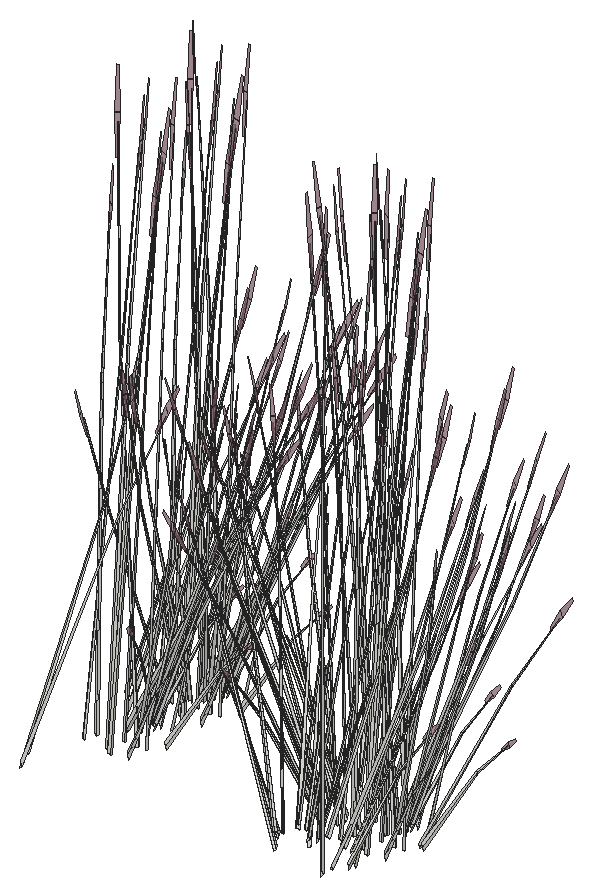
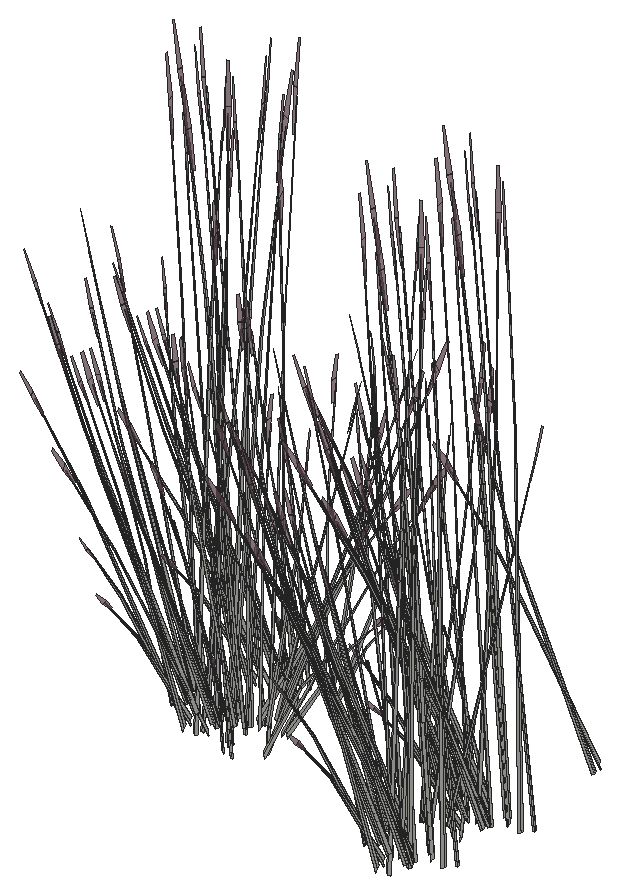
# SketchUp Ruby script. Lengths in inches.
U = 1.inch
M = Sketchup.active_model
def pt(a) = Geom::Point3d.new(a.map { |v| v * U })
def face(e, loops, mat)
  f = e.add_face(loops[0].map { |a| pt(a) })
  loops[1..].each { |l| e.add_face(l.map { |a| pt(a) }).erase! }
  f.material = f.back_material = mat if mat
  f
end
# faces: each face lists its corners as indices into pts; further lists are holes
def faces(e, pts, list, mat = nil) = list.each { |f| face(e, (f[0].is_a?(Array) ? f : [f]).map { |l| l.map { |i| pts[i] } }, mat) }
# xy, xz, yz: faces in a plane at the given z, y or x. An outline is a flat list of corners, or four numbers for a rectangle; further outlines are holes
def ring(l) = l.size == 4 ? [[l[0], l[1]], [l[2], l[1]], [l[2], l[3]], [l[0], l[3]]] : l.each_slice(2).to_a
def flat(e, list, mat, &to3) = list.each { |f| face(e, (f[0].is_a?(Array) ? f : [f]).map { |l| ring(l).map { |u, v| to3.(u, v) } }, mat) }
def xy(e, z, list, mat = nil) = flat(e, list, mat) { |x, y| [x, y, z] }
def xz(e, y, list, mat = nil) = flat(e, list, mat) { |x, z| [x, y, z] }
def yz(e, x, list, mat = nil) = flat(e, list, mat) { |y, z| [x, y, z] }
def lines(e, pts, list) = list.each { |a, b| e.add_line(pt(pts[a]), pt(pts[b])) }
# prism: a flat outline (further loops are holes) pulled along v
def prism(e, loops, v, mat = nil)
  f = face(e, loops, mat); d = Geom::Vector3d.new(v.map { |x| x * U })
  f.pushpull(f.normal.samedirection?(d) ? d.length : -d.length)
end
def box(e, o, s, mat = nil) = prism(e, [[o, [o[0] + s[0], o[1], o[2]], [o[0] + s[0], o[1] + s[1], o[2]], [o[0], o[1] + s[1], o[2]]]], [0, 0, s[2]], mat)
def at(x, y, z, deg = 0) = Geom::Transformation.translation(pt([x, y, z])) * Geom::Transformation.rotation(ORIGIN, Z_AXIS, deg.degrees)
def axes(o, x, y, z) = Geom::Transformation.new([*x, 0, *y, 0, *z, 0, *pt(o).to_a, 1])
def part(name) = M.definitions.add(name)
# library, detail: a bought-in or finely detailed component or shape, given as its bounding box
def library(name, o, s) = part(name).tap { |d| box(d.entities, o, s) }
def detail(e, o, s) = box(e.add_group.entities, o, s)
def put(e, d, t, mat = nil) = e.add_instance(d, t).tap { |i| i.material = mat if mat }
def group(e, t, mat = nil) = e.add_group.tap { |g| g.transformation = t; g.material = mat if mat }.entities
root = M.entities
M.materials.add("LightPink_Translucent").color = [144, 107, 117]
M.materials["LightPink_Translucent"].alpha = 0.75
c1 = part("blade")
p = [[2.15,0.21,22],[0,0.17,0],[0.09,0.45,0],[2.18,0.31,22],[2.29,0.31,22],[0.38,0.45,0],
  [2.48,0.24,33],[2.49,0.24,33],[2.48,0.22,33]]
faces(c1.entities,p,[[0,1,2,3],[4,5,2,3],[6,3,4,7],[8,0,3,6]])
c2 = part("seeds")
p = [[0.3,-0.1,1.38],[-0.01,-0.03,1.59],[-0.01,-0.03,0.03],[0.14,-0.07,-0.07],[0.29,-0.03,3],[0.15,0.01,3.11]]
faces(c2.entities,p,[[0,1,2,3],[1,0,4,5]],"LightPink_Translucent")
c3 = part("blade with seeds")
put(c3.entities,c1,at(0,0,0))
put(c3.entities,c2,axes([2.4,0.25,30.99],[1.5799,-0.05474,1.17369],[-0.12525,1.92788,0.29478],[-0.07173,-0.02425,1.56792]))
put(root,c3,axes([695.78,337.4,512.15],[0.2261,0.04687,1.18691],[0.14573,0.47875,-0.25526],[-0.30712,0.08962,0.50747]))
put(root,c3,axes([676.98,335.32,513.89],[0.63954,0.14313,-0.42412],[-0.21921,0.49074,-0.32852],[0.05864,0.19758,0.81151]))
put(root,c3,axes([677.34,334.31,513.22],[-0.14872,-0.18332,1.42242],[0.6872,-0.15433,0.11501],[0.15531,0.28779,0.60807]))
put(root,c3,axes([681.42,340.66,512.3],[-0.2167,0.29065,0.95334],[-0.18626,-0.3905,0.70045],[0.17898,-0.09785,0.20998]))
put(root,c3,axes([702.6,340.66,512.3],[-0.2167,0.29065,0.95334],[-0.18626,-0.3905,0.70045],[0.17898,-0.09785,0.20998]))
put(root,c3,axes([695.3,338.41,512.3],[0.27113,-0.25877,0.95334],[0.10699,0.40966,0.70045],[-0.19594,0.07335,0.20998]))
put(root,c3,axes([701.83,337.93,513.76],[0.37017,0.35748,-0.29394],[-0.42268,0.3384,0.37948],[0.21476,0.05149,0.72609]))
put(root,c3,axes([681.11,341.75,513.76],[0.56631,-0.0816,-0.29394],[0.14954,0.46647,0.37948],[0.16229,-0.12529,0.72609]))
put(root,c3,axes([702.29,341.75,513.76],[0.56631,-0.0816,-0.29394],[0.14954,0.46647,0.37948],[0.16229,-0.12529,0.72609]))
put(root,c3,axes([696.33,337.29,513.76],[-0.56631,0.0816,-0.29394],[-0.14954,-0.46647,0.37948],[-0.16229,0.12529,0.72609]))
put(root,c3,axes([696.78,341.11,513.76],[-0.37017,-0.35748,-0.29394],[0.42268,-0.3384,0.37948],[-0.21476,-0.05149,0.72609]))
put(root,c3,axes([696.65,341.49,512.15],[0.12702,0.15896,1.18691],[-0.2927,0.4321,-0.25526],[-0.30054,-0.10328,0.50747]))
put(root,c3,axes([697.17,341.35,514.13],[-0.65035,-0.01375,-0.58968],[0.04368,-0.5789,0.07116],[-0.27552,-0.06109,0.83415]))
put(root,c3,axes([701.4,338.13,512.3],[-0.36631,-0.16417,0.95334],[0.47299,-0.16681,0.70045],[0.12758,0.1413,0.20998]))
put(root,c3,axes([696.79,337.34,513.89],[0.16713,0.52135,-0.42412],[-0.63294,0.0912,-0.32852],[-0.18138,0.14003,0.81151]))
put(root,c3,axes([700.5,336.29,512.36],[-0.01777,-0.53759,1.17256],[0.80434,0.13935,0.49647],[-0.19024,0.29416,1.1068]))
put(root,c3,axes([696.96,341.46,513.89],[-0.47241,0.37822,-0.42412],[-0.41372,-0.39954,-0.32852],[-0.24002,-0.05755,0.81151]))
put(root,c3,axes([700.57,338.36,513.89],[0.64198,-0.13573,-0.42412],[0.1123,0.514,-0.32852],[0.17243,0.1473,0.81151]))
put(root,c3,axes([695.89,341.96,512.3],[0.41536,-0.04086,0.95334],[-0.26347,0.35999,0.70045],[-0.20525,-0.054,0.20998]))
put(root,c3,axes([677.66,342.3,512.26],[-0.70648,0.03525,0.37133],[-0.06389,-0.58508,-0.17871],[0.12647,-0.0593,1.19224]))
put(root,c3,axes([698.83,342.3,512.26],[-0.70648,0.03525,0.37133],[-0.06389,-0.58508,-0.17871],[0.12647,-0.0593,1.19224]))
put(root,c3,axes([697.01,342.72,512.06],[0,0.57097,0.4121],[-0.72788,0,0],[0,-0.13004,1.30728]))
put(root,c3,axes([701.45,338.88,512.21],[-0.4172,-0.01791,0.872],[0.27552,-0.38032,0.48145],[0.16481,0.13512,0.68401]))
put(root,c3,axes([680.94,342.85,513.89],[0.17625,-0.51936,-0.42412],[0.60429,0.17802,-0.32852],[0.2433,-0.04762,0.81151]))
put(root,c3,axes([702.11,342.85,513.89],[0.17625,-0.51936,-0.42412],[0.60429,0.17802,-0.32852],[0.2433,-0.04762,0.81151]))
put(root,c3,axes([698.66,343.01,512.26],[-0.31565,0.51449,0.37133],[-0.65588,-0.24761,-0.17871],[0,-0.1186,1.19224]))
put(root,c3,axes([679.64,341.04,512.06],[-0.60889,-0.28548,0.4121],[0.36394,-0.51192,0],[0.13868,0.06502,1.30728]))
put(root,c3,axes([700.81,341.04,512.06],[-0.60889,-0.28548,0.4121],[0.36394,-0.51192,0],[0.13868,0.06502,1.30728]))
put(root,c3,axes([680.83,343.04,514.13],[0.57168,-0.25217,-0.58968],[0.3186,0.51908,0.07116],[0.27622,-0.05897,0.83415]))
put(root,c3,axes([702,343.04,514.13],[0.57168,-0.25217,-0.58968],[0.3186,0.51908,0.07116],[0.27622,-0.05897,0.83415]))
put(root,c3,axes([700.09,337.96,512.15],[0.01148,-0.18927,1.18691],[0.54864,-0.21141,-0.25526],[0.16937,0.22654,0.50747]))
put(root,c3,axes([697.32,338.37,513.76],[-0.4402,0.30062,-0.29394],[-0.41671,-0.34326,0.37948],[-0.0634,0.1744,0.72609]))
put(root,c3,axes([697.6,339.54,512.3],[-0.01684,-0.3395,0.95334],[0.42072,0.24214,0.70045],[-0.08274,0.16182,0.20998]))
put(root,c3,axes([677.33,341.29,512.05],[-0.18794,0.56744,0.14643],[-0.68774,-0.16058,0.29122],[0.1188,-0.00276,1.33138]))
put(root,c3,axes([698.5,341.29,512.05],[-0.18794,0.56744,0.14643],[-0.68774,-0.16058,0.29122],[0.1188,-0.00276,1.33138]))
put(root,c3,axes([678.5,342.06,512.26],[-0.39083,-0.47924,0.37133],[0.59199,-0.33747,-0.17871],[0.12647,0.0593,1.19224]))
put(root,c3,axes([699.67,342.06,512.26],[-0.39083,-0.47924,0.37133],[0.59199,-0.33747,-0.17871],[0.12647,0.0593,1.19224]))
put(root,c3,axes([697.76,338.23,514.15],[0.46573,0.38364,-0.47077],[-0.49199,0.33598,-0.36465],[-0.07086,0.19492,0.90078]))
put(root,c3,axes([699.14,338.6,513.89],[0.63954,0.14313,-0.42412],[-0.21921,0.49074,-0.32852],[0.05864,0.19758,0.81151]))
put(root,c3,axes([680.78,347.32,514.13],[0.01693,-0.52814,-0.58968],[0.71285,0.03547,0.07116],[0.07523,-0.22375,0.83415]))
put(root,c3,axes([698.43,344.22,512.05],[0.6991,-0.15154,0.14643],[0.17263,0.56398,0.29122],[-0.06235,-0.08217,1.33138]))
put(root,c3,axes([681.3125,343.09,513.76],[0.54068,0.15928,-0.29394],[-0.1577,0.46469,0.37948],[0.21769,-0.04261,0.72609]))
put(root,c3,axes([702.48,343.09,513.76],[0.54068,0.15928,-0.29394],[-0.1577,0.46469,0.37948],[0.21769,-0.04261,0.72609]))
put(root,c3,axes([679.54,346.47,513.76],[0.19614,-0.43908,-0.29394],[0.57222,0.12807,0.37948],[-0.05247,-0.17678,0.72609]))
put(root,c3,axes([679.97,347.05,513.22],[-0.12114,0.19625,1.42242],[-0.50818,-0.40613,0.11501],[0.22925,-0.25313,0.60807]))
put(root,c3,axes([698.85,338.9,513.76],[-0.19614,0.43908,-0.29394],[-0.57222,-0.12807,0.37948],[0.05247,0.17678,0.72609]))
put(root,c3,axes([696.13,342.35,513.76],[-0.54068,-0.15928,-0.29394],[0.1577,-0.46469,0.37948],[-0.21769,0.04261,0.72609]))
put(root,c3,axes([697.62,338.05,514.43],[-0.01693,0.52814,-0.65454],[-0.71285,-0.03547,0.07899],[-0.07523,0.22375,0.92591]))
put(root,c3,axes([679.64,345.54,512.3],[0.08346,0.33295,0.95334],[-0.46298,-0.1844,0.70045],[0.04982,-0.17048,0.20998]))
put(root,c3,axes([679.41,341.32,512.05],[-0.6991,0.15154,0.14643],[-0.17263,-0.56398,0.29122],[0.06235,0.08217,1.33138]))
put(root,c3,axes([700.58,341.32,512.05],[-0.6991,0.15154,0.14643],[-0.17263,-0.56398,0.29122],[0.06235,0.08217,1.33138]))
put(root,c3,axes([680.63,347.14,513.89],[-0.46573,-0.38364,-0.42412],[0.49199,-0.33598,-0.32852],[0.07086,-0.19492,0.81151]))
put(root,c3,axes([679.84,342.51,513.22],[-0.26985,0.01293,1.42242],[0.17902,-0.56047,0.11501],[0.38456,0.03467,0.60807]))
put(root,c3,axes([698.91,338.5,514.13],[0.31051,0.46426,-0.58968],[-0.63919,0.25873,0.07116],[0.07261,0.22432,0.83415]))
put(root,c3,axes([697.11,339.24,512.15],[0.2053,-0.09007,1.18691],[0.50689,0.27159,-0.25526],[-0.15087,0.235,0.50747]))
put(root,c3,axes([681.07,347,513.76],[0.4402,-0.30062,-0.29394],[0.41671,0.34326,0.37948],[0.0634,-0.1744,0.72609]))
put(root,c3,axes([700.51,344.25,512.05],[0.18794,-0.56744,0.14643],[0.68774,0.16058,0.29122],[-0.1188,0.00276,1.33138]))
put(root,c3,axes([697.78,342.27,512.77],[0.18493,-0.0826,1.46963],[0.06377,0.5767,0.11501],[-0.40056,0.07652,0.52526]))
put(root,c3,axes([680.41,342.8,512.05],[-0.51116,-0.4159,0.14643],[0.51512,-0.4034,0.29122],[-0.05645,0.08494,1.33138]))
put(root,c3,axes([701.59,342.8,512.05],[-0.51116,-0.4159,0.14643],[0.51512,-0.4034,0.29122],[-0.05645,0.08494,1.33138]))
put(root,c3,axes([682.46,343.18,512.3],[-0.40197,0.09426,0.95334],[0.18921,-0.38956,0.70045],[0.21325,0.02666,0.20998]))
put(root,c3,axes([703.63,343.18,512.3],[-0.40197,0.09426,0.95334],[0.18921,-0.38956,0.70045],[0.21325,0.02666,0.20998]))
put(root,c3,axes([698.21,344.51,512.06],[0.60889,0.28548,0.4121],[-0.36394,0.51192,0],[-0.13868,-0.06502,1.30728]))
put(root,c3,axes([679.18,342.53,512.26],[0.31565,-0.51449,0.37133],[0.65588,0.24761,-0.17871],[0,0.1186,1.19224]))
put(root,c3,axes([700.35,342.53,512.26],[0.31565,-0.51449,0.37133],[0.65588,0.24761,-0.17871],[0,0.1186,1.19224]))
put(root,c3,axes([697.38,338.79,512.79],[0.01429,-0.29475,1.28107],[0.64291,0.15569,0.17703],[-0.0557,0.31414,0.60492]))
put(root,c3,axes([696.5,342.59,513.89],[-0.17625,0.51936,-0.42412],[-0.60429,-0.17802,-0.32852],[-0.2433,0.04762,0.81151]))
put(root,c3,axes([681.76,344.38,513.26],[-0.12452,-0.47997,-0.02898],[0.58854,-0.11034,-0.1314],[0.1229,0.03043,0.43341]))
put(root,c3,axes([702.93,344.38,513.26],[-0.12452,-0.47997,-0.02898],[0.58854,-0.11034,-0.1314],[0.1229,0.03043,0.43341]))
put(root,c3,axes([680.84,342.82,512.06],[0,-0.57097,0.4121],[0.72788,0,0],[0,0.13004,1.30728]))
put(root,c3,axes([702.01,342.82,512.06],[0,-0.57097,0.4121],[0.72788,0,0],[0,0.13004,1.30728]))
put(root,c3,axes([700.18,343.25,512.26],[0.70648,-0.03525,0.37133],[0.06389,0.58508,-0.17871],[-0.12647,0.0593,1.19224]))
put(root,c3,axes([702.88,343.81,512.15],[-0.15668,-0.14043,1.18691],[0.20386,-0.46454,-0.25526],[0.31701,0.06293,0.50747]))
put(root,c3,axes([681.62,348.24,514.13],[0.33983,-0.45051,-0.58968],[0.59551,0.32017,0.07116],[0.20291,-0.16322,0.83415]))
put(root,c3,axes([681.6,348.03,513.89],[-0.16713,-0.52135,-0.42412],[0.63294,-0.0912,-0.32852],[0.18138,-0.14003,0.81151]))
put(root,c3,axes([680.27,344.09,514.13],[0.65035,0.01375,-0.58968],[-0.04368,0.5789,0.07116],[0.27552,0.06109,0.83415]))
put(root,c3,axes([701.44,344.09,514.13],[0.65035,0.01375,-0.58968],[-0.04368,0.5789,0.07116],[0.27552,0.06109,0.83415]))
put(root,c3,axes([700.71,344.55,512.06],[0.60889,-0.28548,0.4121],[0.36394,0.51192,0],[-0.13868,0.06502,1.30728]))
put(root,c3,axes([682.375,346.99,512.3],[-0.2167,0.29065,0.95334],[-0.18626,-0.3905,0.70045],[0.17898,-0.09785,0.20998]))
put(root,c3,axes([695.78,343.8,512.15],[0.2261,0.04687,1.18691],[0.14573,0.47875,-0.25526],[-0.30712,0.08962,0.50747]))
put(root,c3,axes([682.07,348.08,513.76],[0.56631,-0.0816,-0.29394],[0.14954,0.46647,0.37948],[0.16229,-0.12529,0.72609]))
put(root,c3,axes([695.3,344.81,512.3],[0.27113,-0.25877,0.95334],[0.10699,0.40966,0.70045],[-0.19594,0.07335,0.20998]))
put(root,c3,axes([680.66,344.33,513.76],[0.37017,0.35748,-0.29394],[-0.42268,0.3384,0.37948],[0.21476,0.05149,0.72609]))
put(root,c3,axes([701.83,344.33,513.76],[0.37017,0.35748,-0.29394],[-0.42268,0.3384,0.37948],[0.21476,0.05149,0.72609]))
put(root,c3,axes([696.33,343.6875,513.76],[-0.56631,0.0816,-0.29394],[-0.14954,-0.46647,0.37948],[-0.16229,0.12529,0.72609]))
put(root,c3,axes([679.33,343.41,513.22],[-0.24166,-0.09837,1.42242],[0.50011,-0.41269,0.11501],[0.3117,0.18617,0.60807]))
put(root,c3,axes([680.22,344.53,512.3],[-0.36631,-0.16417,0.95334],[0.47299,-0.16681,0.70045],[0.12758,0.1413,0.20998]))
put(root,c3,axes([701.4,344.53,512.3],[-0.36631,-0.16417,0.95334],[0.47299,-0.16681,0.70045],[0.12758,0.1413,0.20998]))
put(root,c3,axes([696.79,343.74,513.89],[0.16713,0.52135,-0.42412],[-0.63294,0.0912,-0.32852],[-0.18138,0.14003,0.81151]))
put(root,c3,axes([700.5,342.6875,512.36],[-0.01777,-0.53759,1.17256],[0.80434,0.13935,0.49647],[-0.19024,0.29416,1.1068]))
put(root,c3,axes([679.4,344.76,513.89],[0.64198,-0.13573,-0.42412],[0.1123,0.514,-0.32852],[0.17243,0.1473,0.81151]))
put(root,c3,axes([700.57,344.76,513.89],[0.64198,-0.13573,-0.42412],[0.1123,0.514,-0.32852],[0.17243,0.1473,0.81151]))
put(root,c3,axes([678.61,348.63,512.26],[-0.70648,0.03525,0.37133],[-0.06389,-0.58508,-0.17871],[0.12647,-0.0593,1.19224]))
put(root,c3,axes([681.89,349.18,513.89],[0.17625,-0.51936,-0.42412],[0.60429,0.17802,-0.32852],[0.2433,-0.04762,0.81151]))
put(root,c3,axes([680.28,345.28,512.21],[-0.4172,-0.01791,0.872],[0.27552,-0.38032,0.48145],[0.16481,0.13512,0.68401]))
put(root,c3,axes([701.45,345.28,512.21],[-0.4172,-0.01791,0.872],[0.27552,-0.38032,0.48145],[0.16481,0.13512,0.68401]))
put(root,c3,axes([680.59,347.37,512.06],[-0.60889,-0.28548,0.4121],[0.36394,-0.51192,0],[0.13868,0.06502,1.30728]))
put(root,c3,axes([681.78,349.37,514.13],[0.57168,-0.25217,-0.58968],[0.3186,0.51908,0.07116],[0.27622,-0.05897,0.83415]))
put(root,c3,axes([700.09,344.36,512.15],[0.01148,-0.18927,1.18691],[0.54864,-0.21141,-0.25526],[0.16937,0.22654,0.50747]))
put(root,c3,axes([697.32,344.77,513.76],[-0.4402,0.30062,-0.29394],[-0.41671,-0.34326,0.37948],[-0.0634,0.1744,0.72609]))
put(root,c3,axes([678.28,347.625,512.05],[-0.18794,0.56744,0.14643],[-0.68774,-0.16058,0.29122],[0.1188,-0.00276,1.33138]))
put(root,c3,axes([697.6,345.9375,512.3],[-0.01684,-0.3395,0.95334],[0.42072,0.24214,0.70045],[-0.08274,0.16182,0.20998]))
put(root,c3,axes([679.45,348.39,512.26],[-0.39083,-0.47924,0.37133],[0.59199,-0.33747,-0.17871],[0.12647,0.0593,1.19224]))
put(root,c3,axes([697.76,344.625,514.15],[0.46573,0.38364,-0.47077],[-0.49199,0.33598,-0.36465],[-0.07086,0.19492,0.90078]))
put(root,c3,axes([677.97,345,513.89],[0.63954,0.14313,-0.42412],[-0.21921,0.49074,-0.32852],[0.05864,0.19758,0.81151]))
put(root,c3,axes([699.14,345,513.89],[0.63954,0.14313,-0.42412],[-0.21921,0.49074,-0.32852],[0.05864,0.19758,0.81151]))
put(root,c3,axes([678.33,343.99,513.22],[-0.14872,-0.18332,1.42242],[0.6872,-0.15433,0.11501],[0.15531,0.28779,0.60807]))
put(root,c3,axes([682.26,349.42,513.76],[0.54068,0.15928,-0.29394],[-0.1577,0.46469,0.37948],[0.21769,-0.04261,0.72609]))
put(root,c3,axes([698.85,345.3,513.76],[-0.19614,0.43908,-0.29394],[-0.57222,-0.12807,0.37948],[0.05247,0.17678,0.72609]))
put(root,c3,axes([680.36,347.66,512.05],[-0.6991,0.15154,0.14643],[-0.17263,-0.56398,0.29122],[0.06235,0.08217,1.33138]))
put(root,c3,axes([697.62,344.45,514.43],[-0.01693,0.52814,-0.65454],[-0.71285,-0.03547,0.07899],[-0.07523,0.22375,0.92591]))
put(root,c3,axes([680.79,348.85,513.22],[-0.26985,0.01293,1.42242],[0.17902,-0.56047,0.11501],[0.38456,0.03467,0.60807]))
put(root,c3,axes([677.74,344.9,514.13],[0.31051,0.46426,-0.58968],[-0.63919,0.25873,0.07116],[0.07261,0.22432,0.83415]))
put(root,c3,axes([698.91,344.9,514.13],[0.31051,0.46426,-0.58968],[-0.63919,0.25873,0.07116],[0.07261,0.22432,0.83415]))
put(root,c3,axes([697.11,345.64,512.15],[0.2053,-0.09007,1.18691],[0.50689,0.27159,-0.25526],[-0.15087,0.235,0.50747]))
put(root,c3,axes([681.37,349.13,512.05],[-0.51116,-0.4159,0.14643],[0.51512,-0.4034,0.29122],[-0.05645,0.08494,1.33138]))
put(root,c3,axes([683.41,349.52,512.3],[-0.40197,0.09426,0.95334],[0.18921,-0.38956,0.70045],[0.21325,0.02666,0.20998]))
put(root,c3,axes([680.13,348.86,512.26],[0.31565,-0.51449,0.37133],[0.65588,0.24761,-0.17871],[0,0.1186,1.19224]))
put(root,c3,axes([697.38,345.19,512.79],[0.01429,-0.29475,1.28107],[0.64291,0.15569,0.17703],[-0.0557,0.31414,0.60492]))
put(root,c3,axes([682.71,350.72,513.26],[-0.12452,-0.47997,-0.02898],[0.58854,-0.11034,-0.1314],[0.1229,0.03043,0.43341]))
put(root,c3,axes([681.79,349.15,512.06],[0,-0.57097,0.4121],[0.72788,0,0],[0,0.13004,1.30728]))
put(root,c3,axes([679.96,349.58,512.26],[0.70648,-0.03525,0.37133],[0.06389,0.58508,-0.17871],[-0.12647,0.0593,1.19224]))
put(root,c3,axes([681.22,350.42,514.13],[0.65035,0.01375,-0.58968],[-0.04368,0.5789,0.07116],[0.27552,0.06109,0.83415]))
put(root,c3,axes([680.49,350.89,512.06],[0.60889,-0.28548,0.4121],[0.36394,0.51192,0],[-0.13868,0.06502,1.30728]))
put(root,c3,axes([681.61,350.66,513.76],[0.37017,0.35748,-0.29394],[-0.42268,0.3384,0.37948],[0.21476,0.05149,0.72609]))
put(root,c3,axes([680.28,349.74,513.22],[-0.24166,-0.09837,1.42242],[0.50011,-0.41269,0.11501],[0.3117,0.18617,0.60807]))
put(root,c3,axes([681.17,350.87,512.3],[-0.36631,-0.16417,0.95334],[0.47299,-0.16681,0.70045],[0.12758,0.1413,0.20998]))
put(root,c3,axes([680.35,351.09,513.89],[0.64198,-0.13573,-0.42412],[0.1123,0.514,-0.32852],[0.17243,0.1473,0.81151]))
put(root,c3,axes([681.23,351.61,512.21],[-0.4172,-0.01791,0.872],[0.27552,-0.38032,0.48145],[0.16481,0.13512,0.68401]))
put(root,c3,axes([678.92,351.33,513.89],[0.63954,0.14313,-0.42412],[-0.21921,0.49074,-0.32852],[0.05864,0.19758,0.81151]))
put(root,c3,axes([679.28,350.32,513.22],[-0.14872,-0.18332,1.42242],[0.6872,-0.15433,0.11501],[0.15531,0.28779,0.60807]))
put(root,c3,axes([678.63,351.63,513.76],[-0.19614,0.43908,-0.29394],[-0.57222,-0.12807,0.37948],[0.05247,0.17678,0.72609]))
put(root,c3,axes([678.6875,351.24,514.13],[0.31051,0.46426,-0.58968],[-0.63919,0.25873,0.07116],[0.07261,0.22432,0.83415]))
